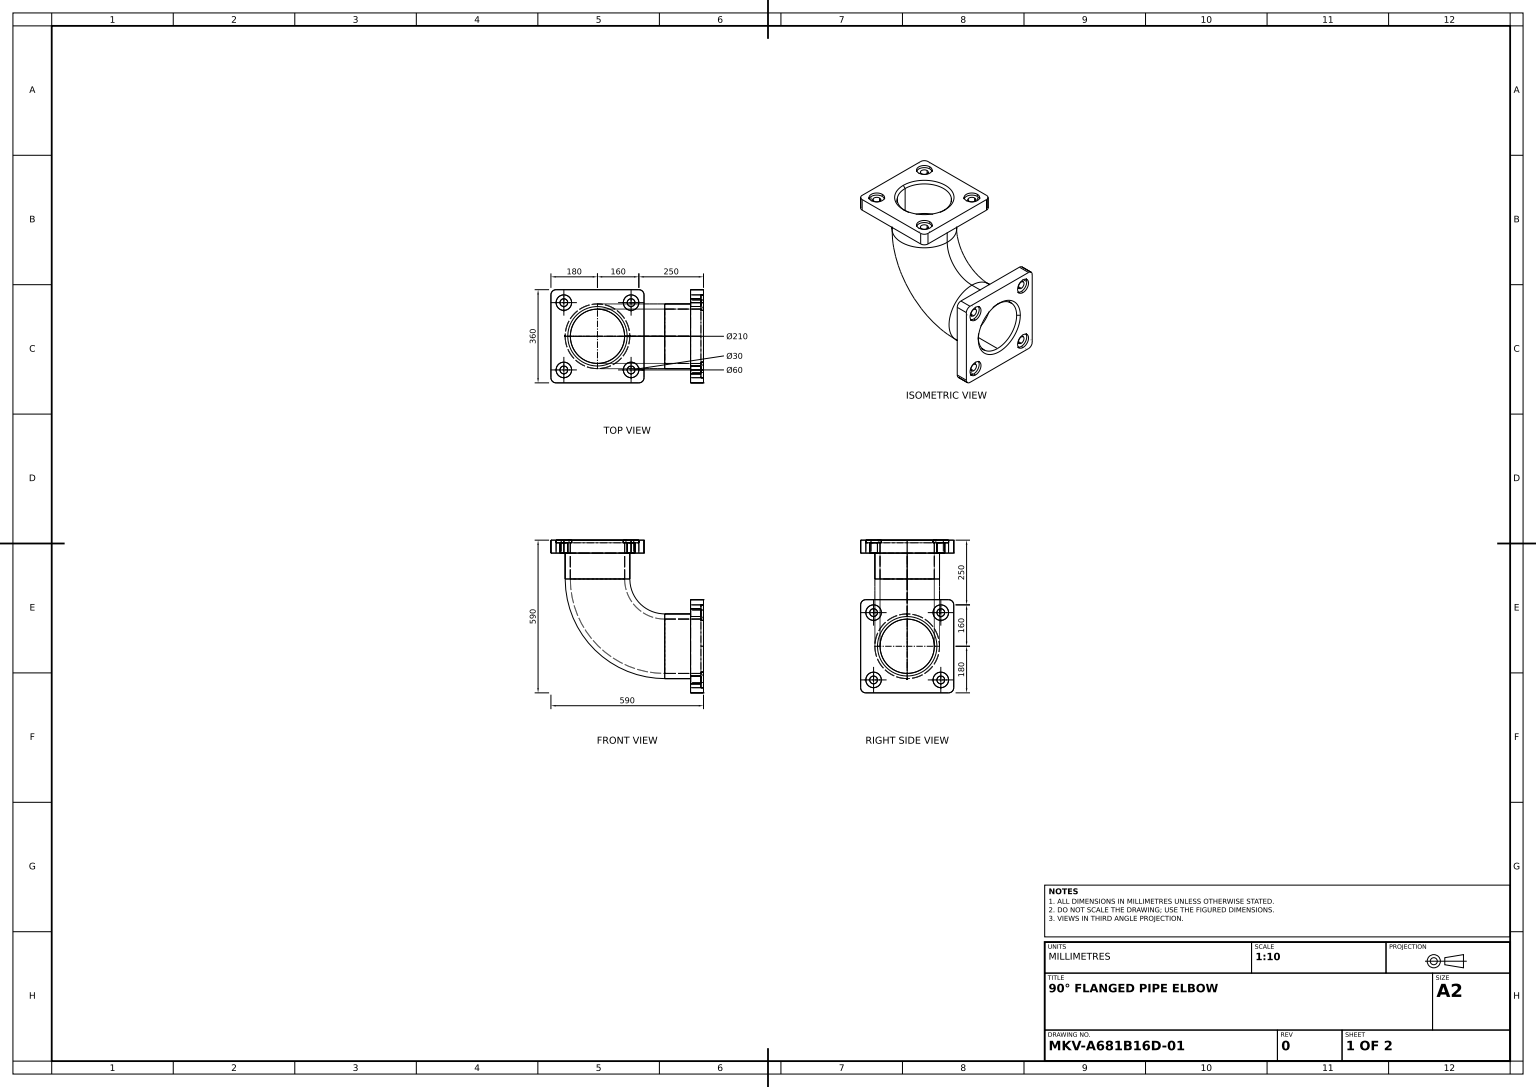
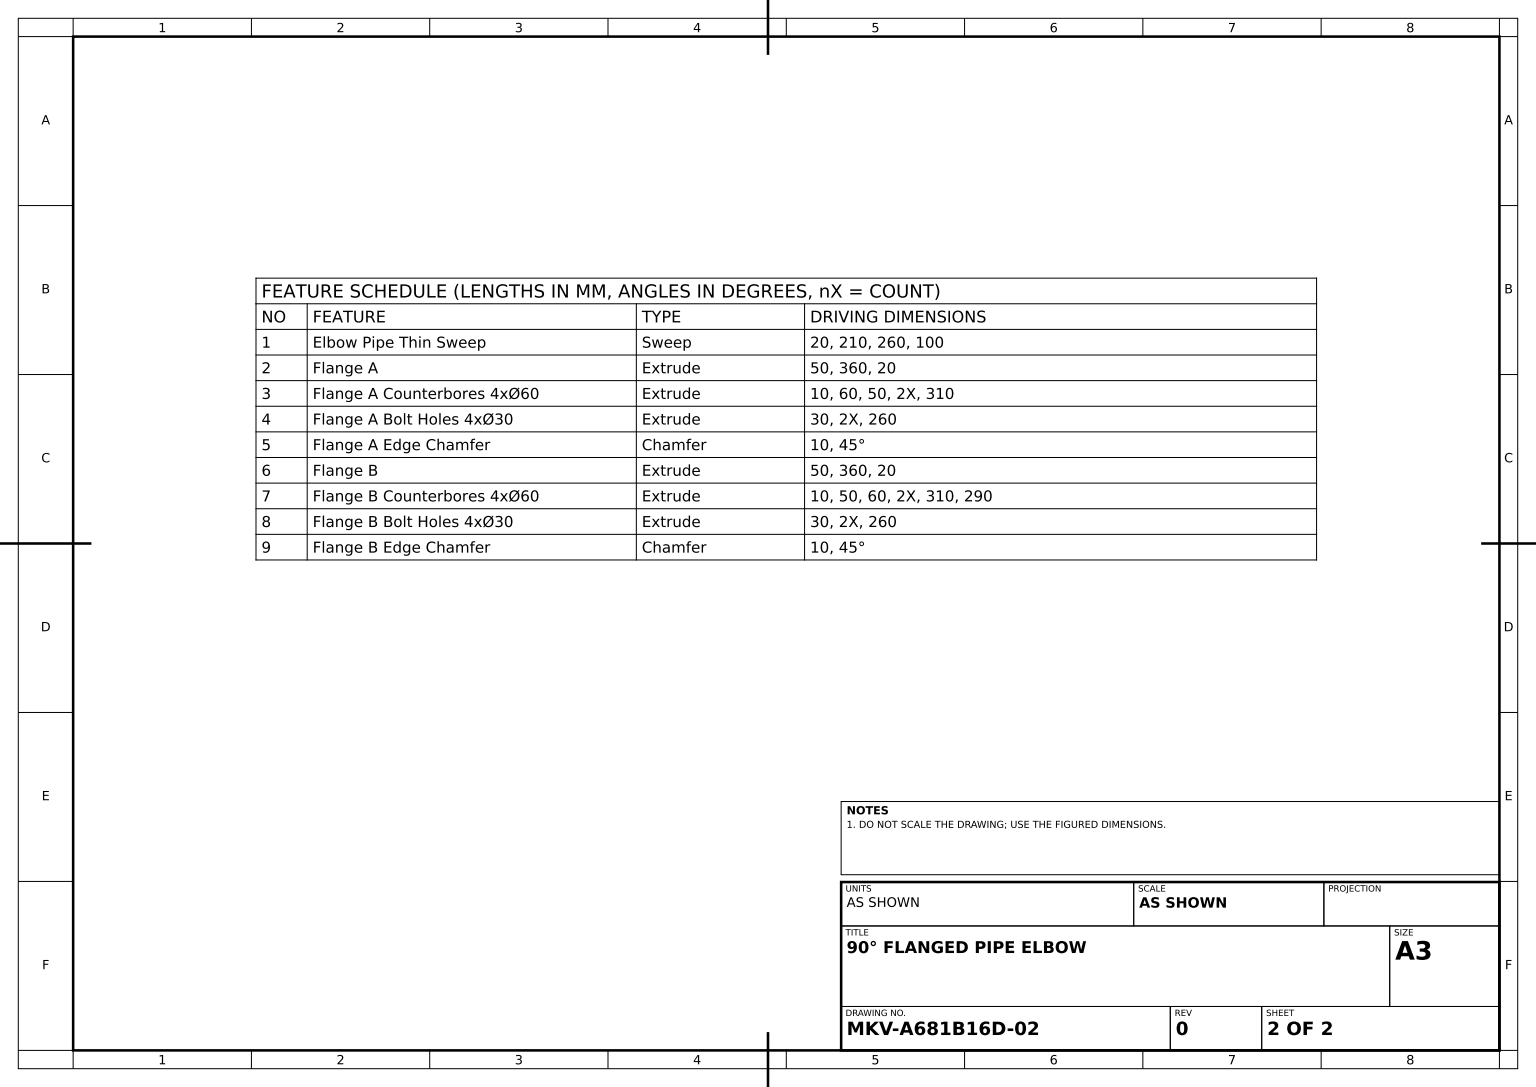
solid
v1 (260,-255,0)
v2 (400,-255,0)
e1 v1 v2 LINE
v3 (400,-360,105)
e2 v2 v3 CIRCLE(AX(P(400,-360,0),D(1,0,0),D(0,0,1)),105)
v4 (400,-465,0)
e3 v3 v4 CIRCLE(AX(P(400,-360,0),D(1,0,0),D(0,0,1)),105)
v5 (260,-465,0)
e4 v5 v4 LINE
e5 v5 v1 CIRCLE(AX(P(260,-360,0),D(-1,0,0),D(0,0,1)),105)
face CYL(AX(P(260,-360,0),D(1,0,0),D(0,1,0)),105) rev [e1 e2 e3 -e4 e5]
v6 (125,-100,0)
v7 (260,-235,0)
e6 v6 v7 CIRCLE(AX(P(260,-100,0),D(0,0,1),D(1,0,0)),135)
v8 (-125,-100,0)
e7 v8 v6 CIRCLE(AX(P(0,-100,0),D(0,1,0),D(1,0,0)),125)
v9 (260,-485,0)
e8 v8 v9 CIRCLE(AX(P(260,-100,0),D(0,0,1),D(1,0,0)),385)
e9 v9 v7 CIRCLE(AX(P(260,-360,0),D(-1,0,0),D(0,-1,0)),125)
face TORUS(AX(P(260,-100,0),D(0,0,1),D(1,0,0)),260,125) [-e6 -e7 e8 e9]
v10 (410,-520,130)
v11 (410,-460,130)
e10 v10 v11 CIRCLE(AX(P(410,-490,130),D(1,0,0),D(0,1,0)),30)
v12 (400,-460,130)
e11 v12 v11 LINE
v13 (400,-520,130)
e12 v13 v12 CIRCLE(AX(P(400,-490,130),D(1,0,0),D(0,1,0)),30)
e13 v13 v10 LINE
face CYL(AX(P(400,-490,130),D(1,0,0),D(0,1,0)),30) rev [e10 -e11 -e12 e13]
v14 (360,-475,-130)
v15 (360,-505,-130)
e14 v14 v15 CIRCLE(AX(P(360,-490,-130),D(1,0,0),D(0,-1,0)),15)
v16 (400,-475,-130)
e15 v16 v14 LINE
v17 (400,-505,-130)
e16 v17 v16 CIRCLE(AX(P(400,-490,-130),D(-1,0,0),D(0,1,0)),15)
e17 v17 v15 LINE
face CYL(AX(P(410,-490,-130),D(-1,0,0),D(0,-1,0)),15) rev [-e14 -e15 -e16 e17]
v18 (160,50,180)
v19 (160,0,180)
e18 v18 v19 LINE
v20 (-160,50,180)
e19 v20 v18 LINE
v21 (-160,0,180)
e20 v20 v21 LINE
e21 v21 v19 LINE
face PLANE(AX(P(-160,50,180),D(0,0,-1),D(-1,0,0))) rev [-e18 -e19 e20 e21]
v22 (400,-360,-105)
e22 v4 v22 CIRCLE(AX(P(400,-360,0),D(1,0,0),D(0,0,1)),105)
v23 (410,-360,115)
e23 v3 v23 LINE
v24 (410,-360,-115)
e24 v24 v23 CIRCLE(AX(P(410,-360,0),D(-1,0,0),D(0,-1,0)),115)
e25 v22 v24 LINE
face CONE(AX(P(410,-360,0),D(1,0,0),D(0,0,-1)),115,0.785398163) rev [-e22 -e3 e23 -e24 -e25]
v25 (130,50,100)
v26 (130,50,160)
e26 v25 v26 CIRCLE(AX(P(130,50,130),D(0,1,0),D(0,0,1)),30)
e27 v26 v25 CIRCLE(AX(P(130,50,130),D(0,1,0),D(0,0,1)),30)
v27 (-130,50,100)
v28 (-130,50,160)
e28 v27 v28 CIRCLE(AX(P(-130,50,130),D(0,1,0),D(0,0,1)),30)
e29 v28 v27 CIRCLE(AX(P(-130,50,130),D(0,1,0),D(0,0,1)),30)
v29 (-115,50,0)
v30 (115,50,0)
e30 v29 v30 CIRCLE(AX(P(0,50,0),D(0,-1,0),D(0,0,-1)),115)
e31 v30 v29 CIRCLE(AX(P(0,50,0),D(0,-1,0),D(0,0,-1)),115)
v31 (130,50,-160)
v32 (130,50,-100)
e32 v31 v32 CIRCLE(AX(P(130,50,-130),D(0,1,0),D(0,0,1)),30)
e33 v32 v31 CIRCLE(AX(P(130,50,-130),D(0,1,0),D(0,0,1)),30)
v33 (180,50,160)
e34 v18 v33 CIRCLE(AX(P(160,50,160),D(0,1,0),D(0,0,1)),20)
v34 (180,50,-160)
e35 v33 v34 LINE
v35 (160,50,-180)
e36 v34 v35 CIRCLE(AX(P(160,50,-160),D(0,1,0),D(0,0,1)),20)
v36 (-160,50,-180)
e37 v35 v36 LINE
v37 (-180,50,-160)
e38 v36 v37 CIRCLE(AX(P(-160,50,-160),D(0,1,0),D(0,0,-1)),20)
v38 (-180,50,160)
e39 v37 v38 LINE
e40 v38 v20 CIRCLE(AX(P(-160,50,160),D(0,1,0),D(0,0,-1)),20)
v39 (-130,50,-100)
v40 (-130,50,-160)
e41 v39 v40 CIRCLE(AX(P(-130,50,-130),D(0,1,0),D(0,0,1)),30)
e42 v40 v39 CIRCLE(AX(P(-130,50,-130),D(0,1,0),D(0,0,1)),30)
face PLANE(AX(P(-160,50,-160),D(0,-1,0),D(0,0,-1))) rev [-e26 -e27] [-e28 -e29] [e30 e31] [-e32 -e33] [e19 e34 e35 e36 e37 e38 e39 e40] [-e41 -e42]
v41 (-130,0,-145)
v42 (-130,0,-115)
e43 v41 v42 CIRCLE(AX(P(-130,0,-130),D(0,1,0),D(0,0,-1)),15)
e44 v42 v41 CIRCLE(AX(P(-130,0,-130),D(0,1,0),D(0,0,-1)),15)
v43 (125,0,0)
v44 (-125,0,0)
e45 v43 v44 CIRCLE(AX(P(0,0,0),D(0,1,0),D(0,0,1)),125)
e46 v44 v43 CIRCLE(AX(P(0,0,0),D(0,1,0),D(0,0,1)),125)
v45 (-130,0,115)
v46 (-130,0,145)
e47 v45 v46 CIRCLE(AX(P(-130,0,130),D(0,1,0),D(0,0,-1)),15)
e48 v46 v45 CIRCLE(AX(P(-130,0,130),D(0,1,0),D(0,0,-1)),15)
v47 (160,0,-180)
v48 (-160,0,-180)
e49 v47 v48 LINE
v49 (180,0,-160)
e50 v49 v47 CIRCLE(AX(P(160,0,-160),D(0,1,0),D(0,0,1)),20)
v50 (180,0,160)
e51 v50 v49 LINE
e52 v19 v50 CIRCLE(AX(P(160,0,160),D(0,1,0),D(0,0,1)),20)
v51 (-180,0,160)
e53 v51 v21 CIRCLE(AX(P(-160,0,160),D(0,1,0),D(0,0,-1)),20)
v52 (-180,0,-160)
e54 v52 v51 LINE
e55 v48 v52 CIRCLE(AX(P(-160,0,-160),D(0,1,0),D(0,0,-1)),20)
v53 (130,0,-145)
v54 (130,0,-115)
e56 v53 v54 CIRCLE(AX(P(130,0,-130),D(0,1,0),D(0,0,-1)),15)
e57 v54 v53 CIRCLE(AX(P(130,0,-130),D(0,1,0),D(0,0,-1)),15)
v55 (130,0,115)
v56 (130,0,145)
e58 v55 v56 CIRCLE(AX(P(130,0,130),D(0,1,0),D(0,0,-1)),15)
e59 v56 v55 CIRCLE(AX(P(130,0,130),D(0,1,0),D(0,0,-1)),15)
face PLANE(AX(P(-160,0,-160),D(0,-1,0),D(0,0,-1))) [e43 e44] [e45 e46] [e47 e48] [-e49 -e50 -e51 -e52 -e21 -e53 -e54 -e55] [e56 e57] [e58 e59]
v57 (-130,40,100)
v58 (-130,40,160)
e60 v57 v58 CIRCLE(AX(P(-130,40,130),D(0,1,0),D(0,0,1)),30)
e61 v57 v27 LINE
e62 v58 v28 LINE
face CYL(AX(P(-130,40,130),D(0,1,0),D(0,0,1)),30) rev [-e60 e61 e28 -e62]
e63 v33 v50 LINE
e64 v34 v49 LINE
face PLANE(AX(P(180,50,-160),D(-1,0,0),D(0,0,1))) rev [e63 e51 -e64 -e35]
v59 (-130,40,115)
e65 v45 v59 LINE
v60 (-130,40,145)
e66 v59 v60 CIRCLE(AX(P(-130,40,130),D(0,1,0),D(0,0,1)),15)
e67 v46 v60 LINE
face CYL(AX(P(-130,-540.001,130),D(0,1,0),D(0,0,1)),15) rev [-e47 e65 e66 -e67]
v61 (-105,40,0)
v62 (105,40,0)
e68 v61 v62 CIRCLE(AX(P(0,40,0),D(0,1,0),D(1,0,0)),105)
e69 v61 v29 LINE
e70 v62 v30 LINE
face CONE(AX(P(0,40,0),D(0,1,0),D(-1,0,0)),105,0.785398163) rev [-e68 e69 -e31 -e70]
v63 (360,-180,160)
v64 (360,-180,-160)
e71 v63 v64 LINE
v65 (410,-180,160)
e72 v65 v63 LINE
v66 (410,-180,-160)
e73 v65 v66 LINE
e74 v66 v64 LINE
face PLANE(AX(P(410,-180,160),D(0,1,0),D(-1,0,0))) [-e71 -e72 e73 e74]
v67 (410,-520,-180)
v68 (360,-520,-180)
e75 v67 v68 LINE
v69 (410,-540,-160)
e76 v67 v69 CIRCLE(AX(P(410,-520,-160),D(-1,0,0),D(0,-1,0)),20)
v70 (360,-540,-160)
e77 v69 v70 LINE
e78 v68 v70 CIRCLE(AX(P(360,-520,-160),D(-1,0,0),D(0,-1,0)),20)
face CYL(AX(P(410,-520,-160),D(-1,0,0),D(0,-1,0)),20) [-e75 e76 e77 -e78]
v71 (130,40,-145)
v72 (130,40,-115)
e79 v71 v72 CIRCLE(AX(P(130,40,-130),D(0,1,0),D(0,0,1)),15)
e80 v54 v72 LINE
e81 v53 v71 LINE
face CYL(AX(P(130,-540.001,-130),D(0,1,0),D(0,0,1)),15) rev [e79 -e80 -e56 e81]
e82 v1 v5 CIRCLE(AX(P(260,-360,0),D(-1,0,0),D(0,0,1)),105)
v73 (105,-100,0)
e83 v73 v1 CIRCLE(AX(P(260,-100,0),D(0,0,1),D(1,0,0)),155)
v74 (-105,-100,0)
e84 v73 v74 CIRCLE(AX(P(0,-100,0),D(0,1,0),D(0,0,1)),105)
e85 v74 v5 CIRCLE(AX(P(260,-100,0),D(0,0,1),D(1,0,0)),365)
face TORUS(AX(P(260,-100,0),D(0,0,1),D(1,0,0)),260,105) rev [-e82 -e83 e84 e85]
e86 v62 v73 LINE
e87 v62 v61 CIRCLE(AX(P(0,40,0),D(0,1,0),D(1,0,0)),105)
e88 v61 v74 LINE
face CYL(AX(P(0,0,0),D(0,-1,0),D(1,0,0)),105) rev [-e86 e87 e88 -e84]
v75 (400,-505,130)
v76 (360,-505,130)
e89 v75 v76 LINE
v77 (360,-475,130)
e90 v77 v76 CIRCLE(AX(P(360,-490,130),D(1,0,0),D(0,-1,0)),15)
v78 (400,-475,130)
e91 v78 v77 LINE
e92 v75 v78 CIRCLE(AX(P(400,-490,130),D(-1,0,0),D(0,1,0)),15)
face CYL(AX(P(410,-490,130),D(-1,0,0),D(0,-1,0)),15) rev [e89 -e90 -e91 -e92]
e93 v36 v48 LINE
e94 v37 v52 LINE
face CYL(AX(P(-160,50,-160),D(0,-1,0),D(0,0,-1)),20) [-e38 e93 e55 -e94]
e95 v58 v57 CIRCLE(AX(P(-130,40,130),D(0,1,0),D(0,0,1)),30)
face CYL(AX(P(-130,40,130),D(0,1,0),D(0,0,1)),30) rev [e29 -e61 -e95 e62]
e96 v23 v24 CIRCLE(AX(P(410,-360,0),D(-1,0,0),D(0,-1,0)),115)
e97 v22 v2 CIRCLE(AX(P(400,-360,0),D(1,0,0),D(0,0,1)),105)
face CONE(AX(P(410,-360,0),D(1,0,0),D(0,0,-1)),115,0.785398163) rev [e25 -e96 -e23 -e2 -e97]
face CONE(AX(P(0,40,0),D(0,1,0),D(-1,0,0)),105,0.785398163) rev [-e30 -e69 -e87 e70]
v79 (400,-200,130)
v80 (400,-260,130)
e98 v79 v80 CIRCLE(AX(P(400,-230,130),D(1,0,0),D(0,1,0)),30)
v81 (410,-200,130)
e99 v79 v81 LINE
v82 (410,-260,130)
e100 v81 v82 CIRCLE(AX(P(410,-230,130),D(1,0,0),D(0,1,0)),30)
e101 v80 v82 LINE
face CYL(AX(P(400,-230,130),D(1,0,0),D(0,1,0)),30) rev [-e98 e99 e100 -e101]
face CYL(AX(P(160,50,160),D(0,-1,0),D(0,0,-1)),20) [-e34 e18 e52 -e63]
e102 v60 v59 CIRCLE(AX(P(-130,40,130),D(0,1,0),D(0,0,1)),15)
face CYL(AX(P(-130,-540.001,130),D(0,1,0),D(0,0,1)),15) rev [e102 -e65 -e48 e67]
v83 (400,-245,-130)
v84 (400,-215,-130)
e103 v83 v84 CIRCLE(AX(P(400,-230,-130),D(-1,0,0),D(0,1,0)),15)
e104 v84 v83 CIRCLE(AX(P(400,-230,-130),D(-1,0,0),D(0,1,0)),15)
v85 (400,-200,-130)
v86 (400,-260,-130)
e105 v85 v86 CIRCLE(AX(P(400,-230,-130),D(1,0,0),D(0,1,0)),30)
e106 v86 v85 CIRCLE(AX(P(400,-230,-130),D(1,0,0),D(0,1,0)),30)
face PLANE(AX(P(400,-230,-130),D(1,0,0),D(0,1,0))) [e103 e104] [e105 e106]
face CYL(AX(P(260,-360,0),D(1,0,0),D(0,1,0)),105) rev [e82 e4 e22 e97 -e1]
v87 (360,-245,130)
v88 (360,-215,130)
e107 v87 v88 CIRCLE(AX(P(360,-230,130),D(1,0,0),D(0,-1,0)),15)
v89 (400,-245,130)
e108 v89 v87 LINE
v90 (400,-215,130)
e109 v90 v89 CIRCLE(AX(P(400,-230,130),D(-1,0,0),D(0,1,0)),15)
e110 v90 v88 LINE
face CYL(AX(P(410,-230,130),D(-1,0,0),D(0,-1,0)),15) rev [-e107 -e108 -e109 e110]
e111 v78 v75 CIRCLE(AX(P(400,-490,130),D(-1,0,0),D(0,1,0)),15)
e112 v12 v13 CIRCLE(AX(P(400,-490,130),D(1,0,0),D(0,1,0)),30)
face PLANE(AX(P(400,-490,130),D(1,0,0),D(0,1,0))) [e92 e111] [e112 e12]
v91 (-130,40,-100)
e113 v91 v39 LINE
v92 (-130,40,-160)
e114 v92 v91 CIRCLE(AX(P(-130,40,-130),D(0,1,0),D(0,0,1)),30)
e115 v92 v40 LINE
face CYL(AX(P(-130,40,-130),D(0,1,0),D(0,0,1)),30) rev [e42 -e113 -e114 e115]
v93 (360,-235,0)
v94 (360,-485,0)
e116 v93 v94 CIRCLE(AX(P(360,-360,0),D(-1,0,0),D(0,-1,0)),125)
e117 v9 v94 LINE
e118 v7 v9 CIRCLE(AX(P(260,-360,0),D(-1,0,0),D(0,-1,0)),125)
e119 v7 v93 LINE
face CYL(AX(P(260,-360,0),D(1,0,0),D(0,1,0)),125) [e116 -e117 -e118 e119]
v95 (130,40,-100)
e120 v95 v32 LINE
v96 (130,40,-160)
e121 v96 v31 LINE
e122 v95 v96 CIRCLE(AX(P(130,40,-130),D(0,1,0),D(0,0,1)),30)
face CYL(AX(P(130,40,-130),D(0,1,0),D(0,0,1)),30) rev [e120 e33 -e121 -e122]
e123 v11 v10 CIRCLE(AX(P(410,-490,130),D(1,0,0),D(0,1,0)),30)
face CYL(AX(P(400,-490,130),D(1,0,0),D(0,1,0)),30) rev [e11 e123 -e13 -e112]
v97 (360,-245,-130)
e124 v83 v97 LINE
v98 (360,-215,-130)
e125 v84 v98 LINE
e126 v97 v98 CIRCLE(AX(P(360,-230,-130),D(1,0,0),D(0,-1,0)),15)
face CYL(AX(P(410,-230,-130),D(-1,0,0),D(0,-1,0)),15) rev [-e124 -e104 e125 -e126]
e127 v16 v17 CIRCLE(AX(P(400,-490,-130),D(-1,0,0),D(0,1,0)),15)
e128 v15 v14 CIRCLE(AX(P(360,-490,-130),D(1,0,0),D(0,-1,0)),15)
face CYL(AX(P(410,-490,-130),D(-1,0,0),D(0,-1,0)),15) rev [-e17 -e127 e15 -e128]
v99 (410,-260,-130)
v100 (410,-200,-130)
e129 v99 v100 CIRCLE(AX(P(410,-230,-130),D(1,0,0),D(0,1,0)),30)
e130 v85 v100 LINE
e131 v86 v99 LINE
face CYL(AX(P(400,-230,-130),D(1,0,0),D(0,1,0)),30) rev [e129 -e130 -e106 e131]
v101 (130,40,160)
v102 (130,40,100)
e132 v101 v102 CIRCLE(AX(P(130,40,130),D(0,1,0),D(0,0,1)),30)
e133 v101 v26 LINE
e134 v102 v25 LINE
face CYL(AX(P(130,40,130),D(0,1,0),D(0,0,1)),30) rev [-e132 e133 e27 -e134]
e135 v94 v93 CIRCLE(AX(P(360,-360,0),D(-1,0,0),D(0,-1,0)),125)
face CYL(AX(P(260,-360,0),D(1,0,0),D(0,1,0)),125) [e135 -e119 -e9 e117]
v103 (410,-200,180)
v104 (360,-200,180)
e136 v103 v104 LINE
e137 v103 v65 CIRCLE(AX(P(410,-200,160),D(-1,0,0),D(0,-1,0)),20)
e138 v104 v63 CIRCLE(AX(P(360,-200,160),D(-1,0,0),D(0,-1,0)),20)
face CYL(AX(P(410,-200,160),D(-1,0,0),D(0,-1,0)),20) [-e136 e137 e72 -e138]
e139 v98 v97 CIRCLE(AX(P(360,-230,-130),D(1,0,0),D(0,-1,0)),15)
face CYL(AX(P(410,-230,-130),D(-1,0,0),D(0,-1,0)),15) rev [-e103 e124 -e139 -e125]
e140 v43 v6 LINE
e141 v6 v8 CIRCLE(AX(P(0,-100,0),D(0,1,0),D(1,0,0)),125)
e142 v44 v8 LINE
face CYL(AX(P(0,0,0),D(0,-1,0),D(1,0,0)),125) [e140 e141 -e142 -e45]
v105 (400,-520,-130)
v106 (400,-460,-130)
e143 v105 v106 CIRCLE(AX(P(400,-490,-130),D(1,0,0),D(0,1,0)),30)
e144 v106 v105 CIRCLE(AX(P(400,-490,-130),D(1,0,0),D(0,1,0)),30)
face PLANE(AX(P(400,-490,-130),D(1,0,0),D(0,1,0))) [e143 e144] [e16 e127]
e145 v74 v73 CIRCLE(AX(P(0,-100,0),D(0,1,0),D(0,0,1)),105)
face CYL(AX(P(0,0,0),D(0,-1,0),D(1,0,0)),105) rev [-e88 e68 e86 -e145]
v107 (410,-460,-130)
v108 (410,-520,-130)
e146 v107 v108 CIRCLE(AX(P(410,-490,-130),D(1,0,0),D(0,1,0)),30)
e147 v105 v108 LINE
e148 v106 v107 LINE
face CYL(AX(P(400,-490,-130),D(1,0,0),D(0,1,0)),30) rev [e146 -e147 -e144 e148]
v109 (410,-520,180)
e149 v103 v109 LINE
v110 (410,-540,160)
e150 v110 v109 CIRCLE(AX(P(410,-520,160),D(-1,0,0),D(0,-1,0)),20)
e151 v110 v69 LINE
v111 (410,-200,-180)
e152 v111 v67 LINE
e153 v111 v66 CIRCLE(AX(P(410,-200,-160),D(1,0,0),D(0,1,0)),20)
e154 v108 v107 CIRCLE(AX(P(410,-490,-130),D(1,0,0),D(0,1,0)),30)
e155 v82 v81 CIRCLE(AX(P(410,-230,130),D(1,0,0),D(0,1,0)),30)
e156 v100 v99 CIRCLE(AX(P(410,-230,-130),D(1,0,0),D(0,1,0)),30)
face PLANE(AX(P(410,-200,160),D(-1,0,0),D(0,-1,0))) rev [-e73 -e137 e149 -e150 e151 -e76 -e152 e153] [-e10 -e123] [-e154 -e146] [-e155 -e100] [e24 e96] [-e156 -e129]
e157 v102 v101 CIRCLE(AX(P(130,40,130),D(0,1,0),D(0,0,1)),30)
face CYL(AX(P(130,40,130),D(0,1,0),D(0,0,1)),30) rev [e134 e26 -e133 -e157]
e158 v80 v79 CIRCLE(AX(P(400,-230,130),D(1,0,0),D(0,1,0)),30)
e159 v89 v90 CIRCLE(AX(P(400,-230,130),D(-1,0,0),D(0,1,0)),15)
face PLANE(AX(P(400,-230,130),D(1,0,0),D(0,1,0))) [e158 e98] [e109 e159]
e160 v96 v95 CIRCLE(AX(P(130,40,-130),D(0,1,0),D(0,0,1)),30)
e161 v72 v71 CIRCLE(AX(P(130,40,-130),D(0,1,0),D(0,0,1)),15)
face PLANE(AX(P(130,40,-130),D(0,1,0),D(0,0,1))) [e160 e122] [-e79 -e161]
face CYL(AX(P(130,-540.001,-130),D(0,1,0),D(0,0,1)),15) rev [e80 e161 -e81 -e57]
v112 (360,-200,-180)
e162 v111 v112 LINE
e163 v112 v64 CIRCLE(AX(P(360,-200,-160),D(1,0,0),D(0,1,0)),20)
face CYL(AX(P(410,-200,-160),D(-1,0,0),D(0,-1,0)),20) [e162 e163 -e74 -e153]
e164 v35 v47 LINE
face PLANE(AX(P(-160,50,-180),D(0,0,1),D(1,0,0))) rev [e49 -e93 -e37 e164]
face CYL(AX(P(130,40,-130),D(0,1,0),D(0,0,1)),30) rev [e32 -e120 -e160 e121]
e165 v91 v92 CIRCLE(AX(P(-130,40,-130),D(0,1,0),D(0,0,1)),30)
v113 (-130,40,-115)
v114 (-130,40,-145)
e166 v113 v114 CIRCLE(AX(P(-130,40,-130),D(0,1,0),D(0,0,1)),15)
e167 v114 v113 CIRCLE(AX(P(-130,40,-130),D(0,1,0),D(0,0,1)),15)
face PLANE(AX(P(-130,40,-130),D(0,1,0),D(0,0,1))) [e165 e114] [-e166 -e167]
e168 v38 v51 LINE
face PLANE(AX(P(-180,50,-160),D(1,0,0),D(0,0,-1))) rev [e54 -e168 -e39 e94]
e169 v76 v77 CIRCLE(AX(P(360,-490,130),D(1,0,0),D(0,-1,0)),15)
e170 v88 v87 CIRCLE(AX(P(360,-230,130),D(1,0,0),D(0,-1,0)),15)
v115 (360,-540,160)
v116 (360,-520,180)
e171 v115 v116 CIRCLE(AX(P(360,-520,160),D(-1,0,0),D(0,-1,0)),20)
e172 v104 v116 LINE
e173 v112 v68 LINE
e174 v115 v70 LINE
face PLANE(AX(P(360,-200,160),D(-1,0,0),D(0,-1,0))) [e169 e90] [e128 e14] [e170 e107] [e139 e126] [e171 -e172 e138 e71 -e163 e173 e78 -e174] [-e116 -e135]
face CYL(AX(P(400,-230,-130),D(1,0,0),D(0,1,0)),30) rev [-e105 e130 e156 -e131]
face TORUS(AX(P(260,-100,0),D(0,0,1),D(1,0,0)),260,125) [-e8 -e141 e6 e118]
face CYL(AX(P(410,-490,130),D(-1,0,0),D(0,-1,0)),15) rev [-e89 -e111 e91 -e169]
e175 v41 v114 LINE
e176 v42 v113 LINE
face CYL(AX(P(-130,-540.001,-130),D(0,1,0),D(0,0,1)),15) rev [-e43 e175 e167 -e176]
v117 (130,40,145)
v118 (130,40,115)
e177 v117 v118 CIRCLE(AX(P(130,40,130),D(0,1,0),D(0,0,1)),15)
e178 v118 v117 CIRCLE(AX(P(130,40,130),D(0,1,0),D(0,0,1)),15)
face PLANE(AX(P(130,40,130),D(0,1,0),D(0,0,1))) [-e177 -e178] [e132 e157]
face CYL(AX(P(410,-230,130),D(-1,0,0),D(0,-1,0)),15) rev [-e159 e108 -e170 -e110]
e179 v109 v116 LINE
e180 v110 v115 LINE
face CYL(AX(P(410,-520,160),D(-1,0,0),D(0,-1,0)),20) [e150 e179 -e171 -e180]
face PLANE(AX(P(410,-200,180),D(0,0,-1),D(0,1,0))) rev [e136 e172 -e179 -e149]
face PLANE(AX(P(-130,40,130),D(0,1,0),D(0,0,1))) [e60 e95] [-e102 -e66]
face PLANE(AX(P(410,-540,160),D(0,1,0),D(-1,0,0))) rev [-e151 e180 e174 -e77]
face CYL(AX(P(-130,40,-130),D(0,1,0),D(0,0,1)),30) rev [-e165 e113 e41 -e115]
face PLANE(AX(P(410,-200,-180),D(0,0,-1),D(0,1,0))) [e152 e75 -e173 -e162]
face CYL(AX(P(-130,-540.001,-130),D(0,1,0),D(0,0,1)),15) rev [-e44 e176 e166 -e175]
face CYL(AX(P(400,-490,-130),D(1,0,0),D(0,1,0)),30) rev [e147 e154 -e148 -e143]
face CYL(AX(P(160,50,-160),D(0,-1,0),D(0,0,-1)),20) [e64 e50 -e164 -e36]
face CYL(AX(P(400,-230,130),D(1,0,0),D(0,1,0)),30) rev [-e99 -e158 e101 e155]
face TORUS(AX(P(260,-100,0),D(0,0,1),D(1,0,0)),260,105) rev [e145 e83 -e5 -e85]
face CYL(AX(P(0,0,0),D(0,-1,0),D(1,0,0)),125) [e142 e7 -e140 -e46]
face CYL(AX(P(-160,50,160),D(0,-1,0),D(0,0,-1)),20) [-e40 e168 e53 -e20]
e181 v56 v117 LINE
e182 v55 v118 LINE
face CYL(AX(P(130,-540.001,130),D(0,1,0),D(0,0,1)),15) rev [e181 e177 -e182 -e59]
face CYL(AX(P(130,-540.001,130),D(0,1,0),D(0,0,1)),15) rev [-e58 e182 e178 -e181]
